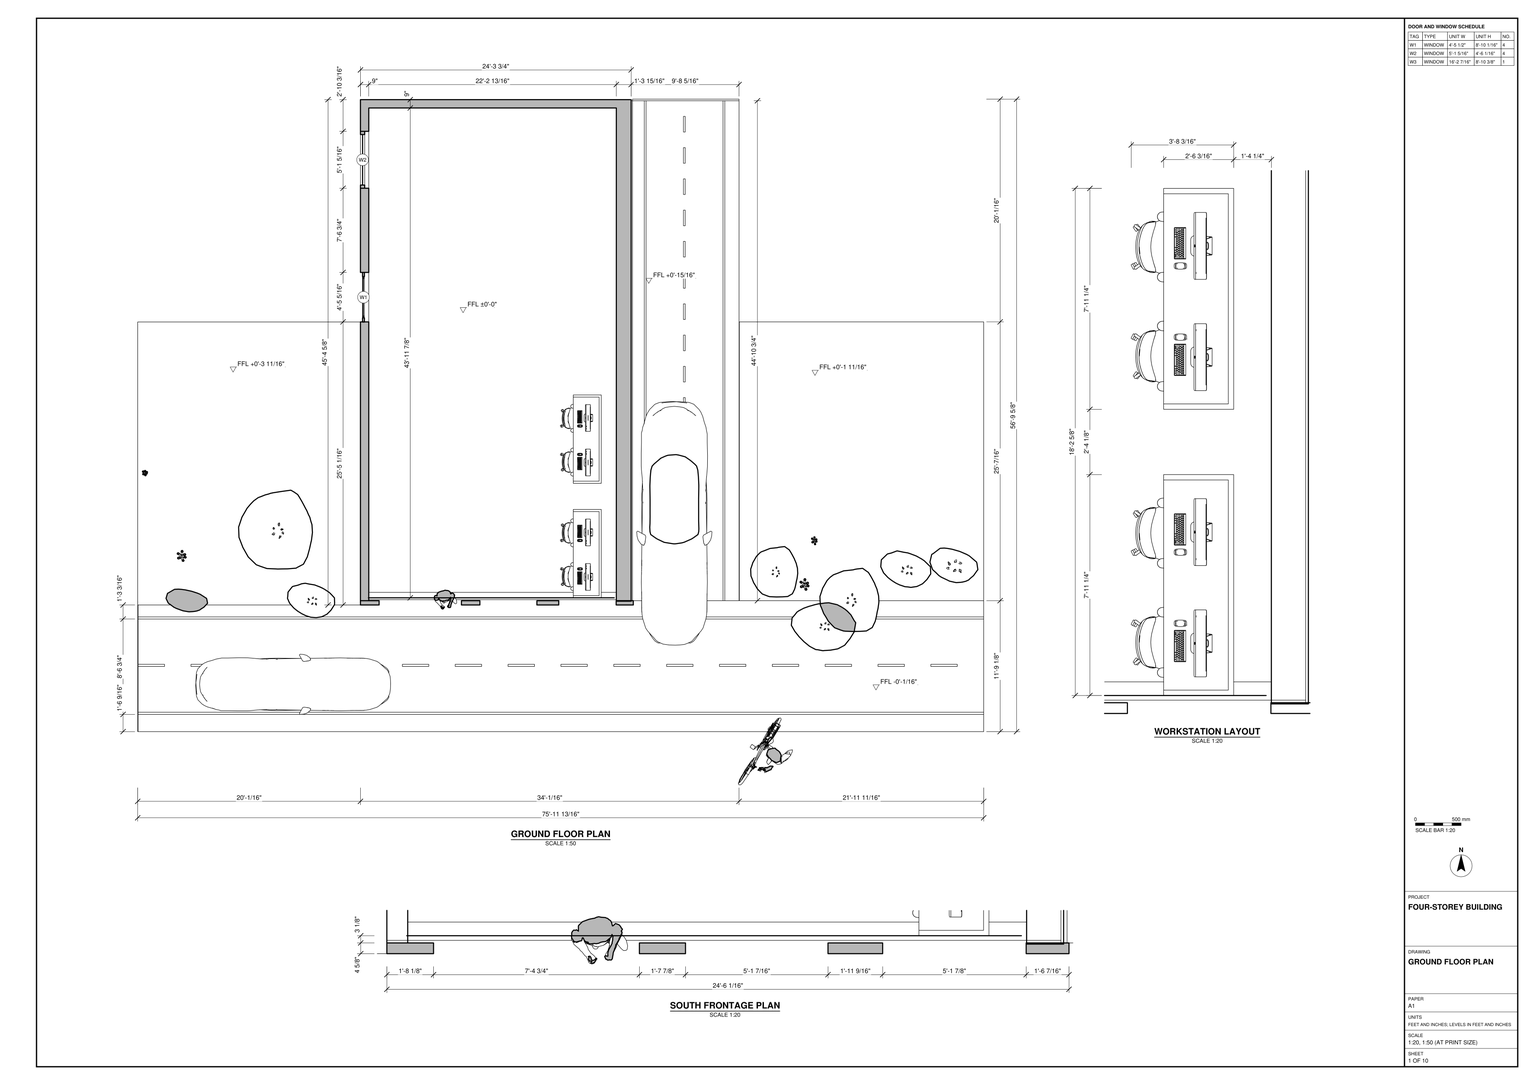
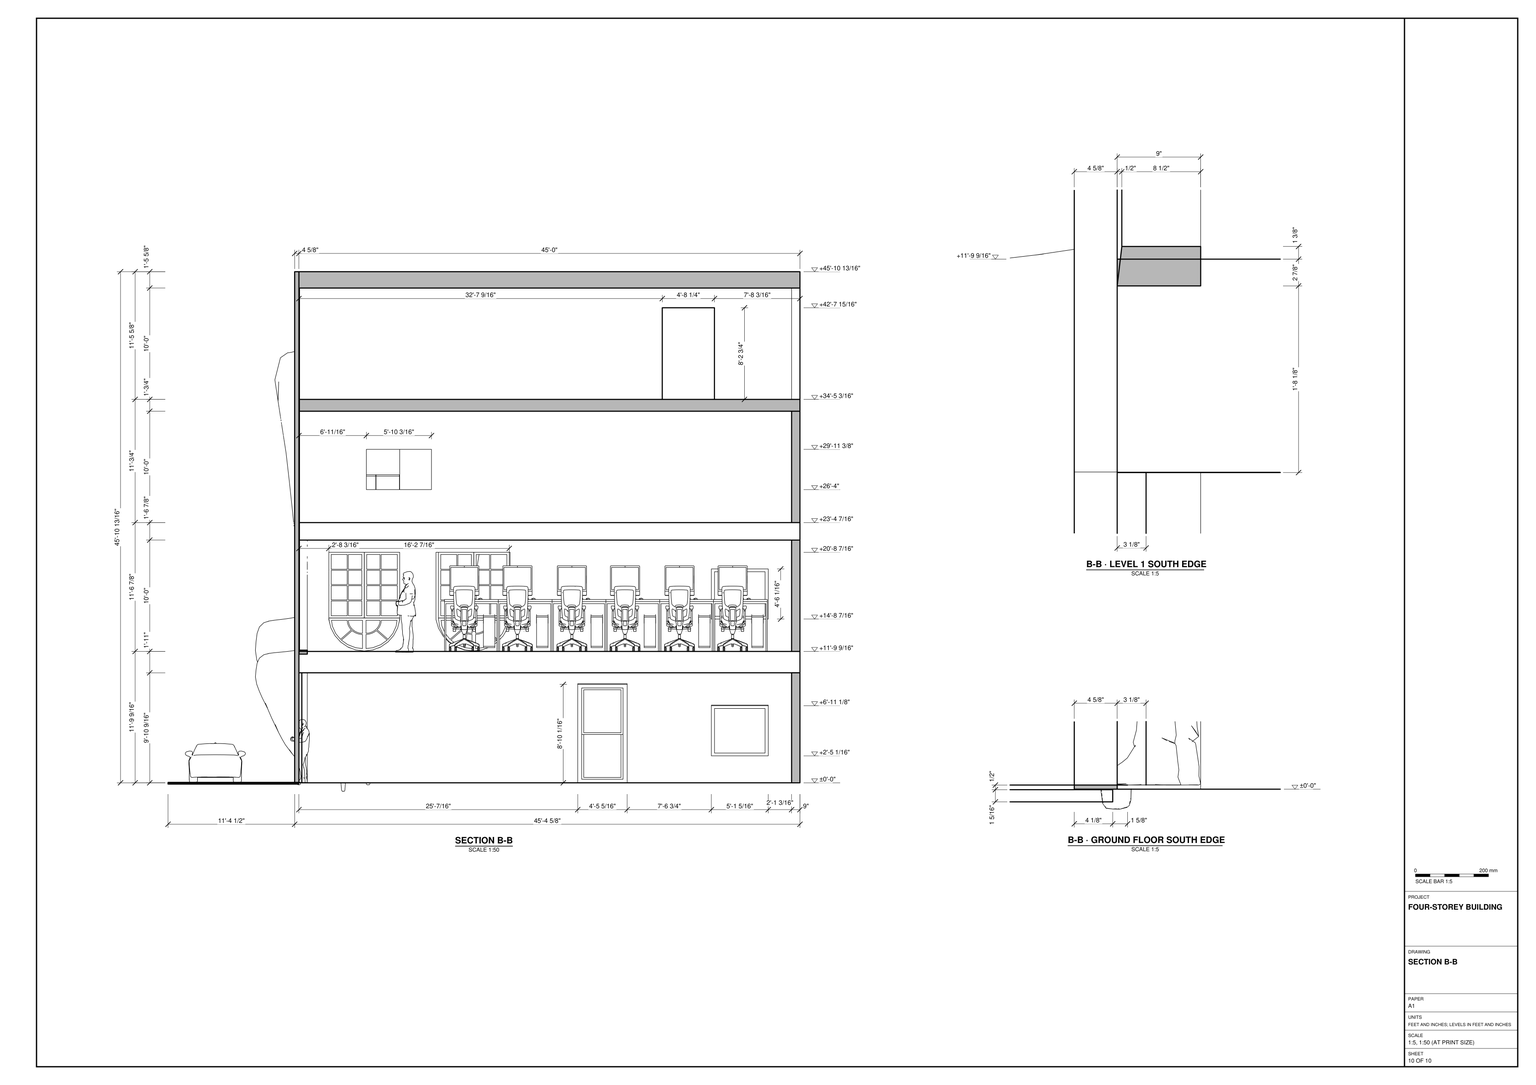
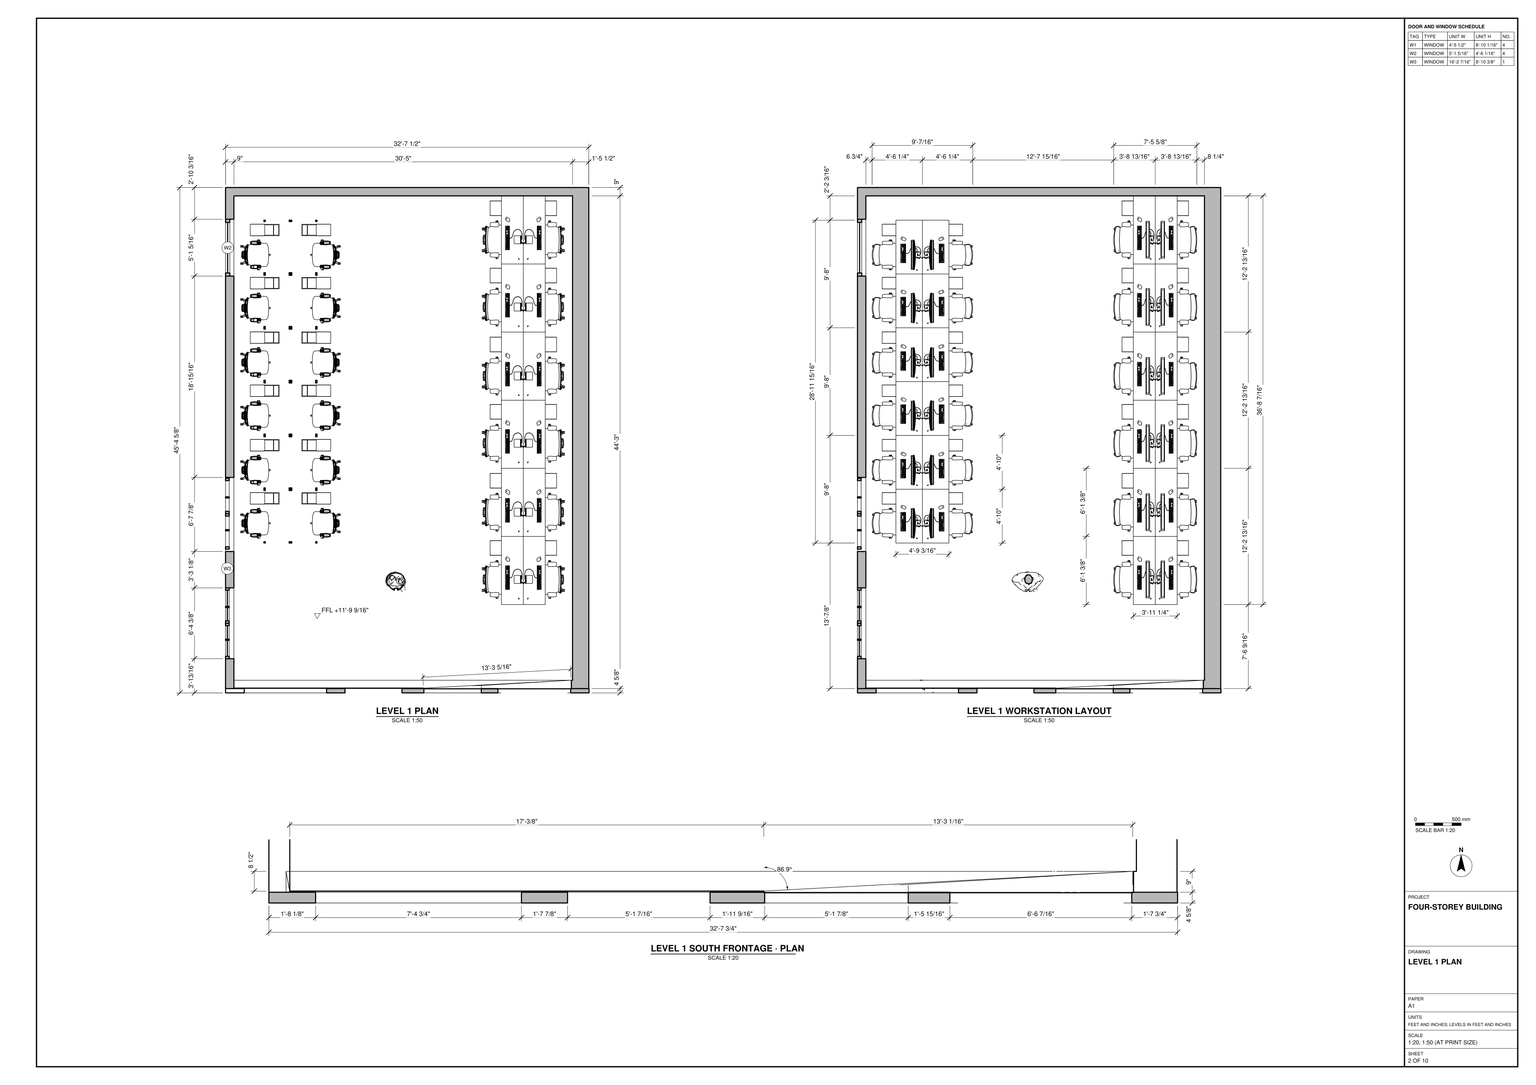
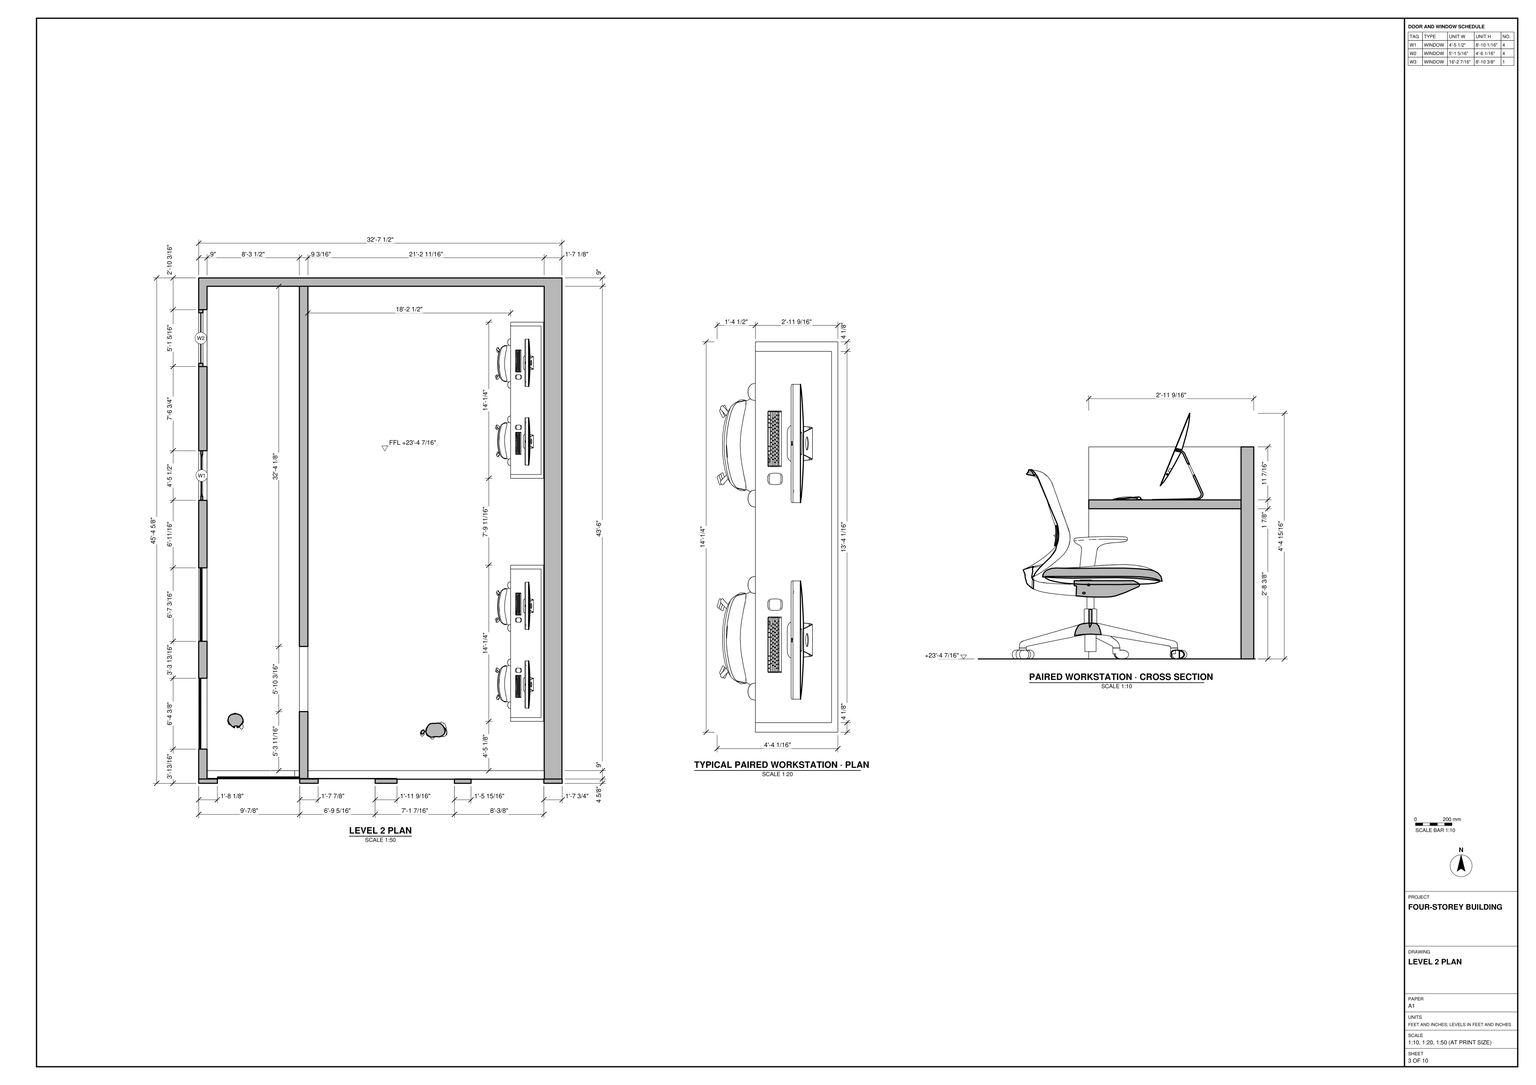
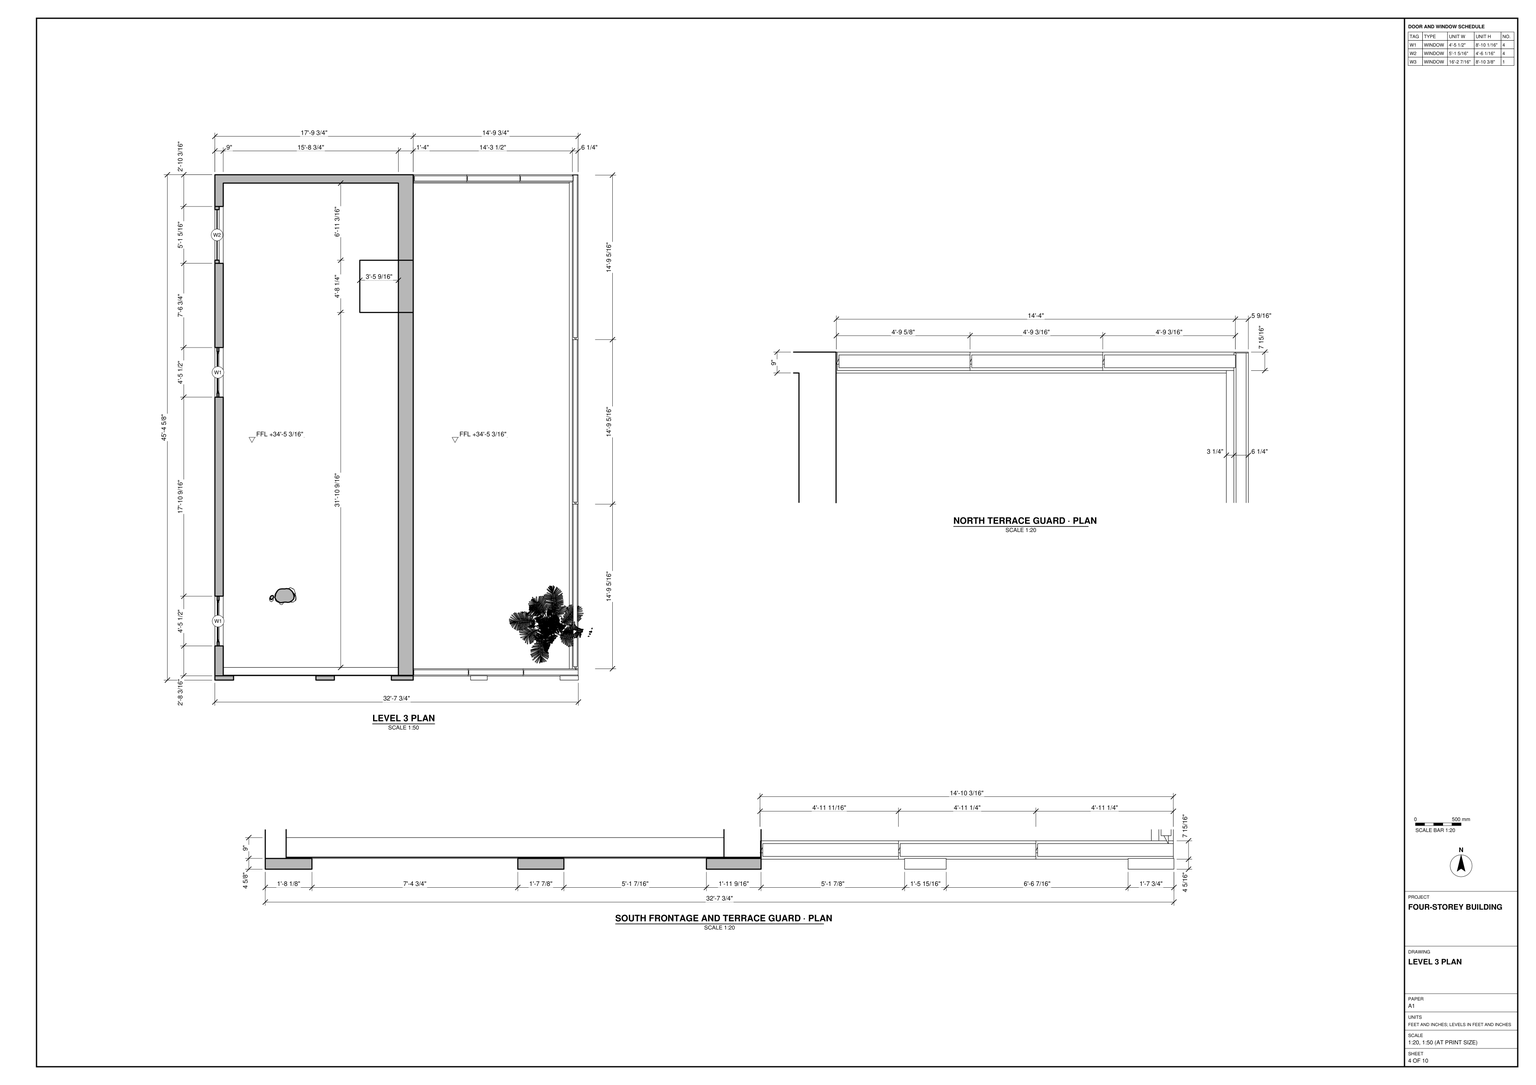
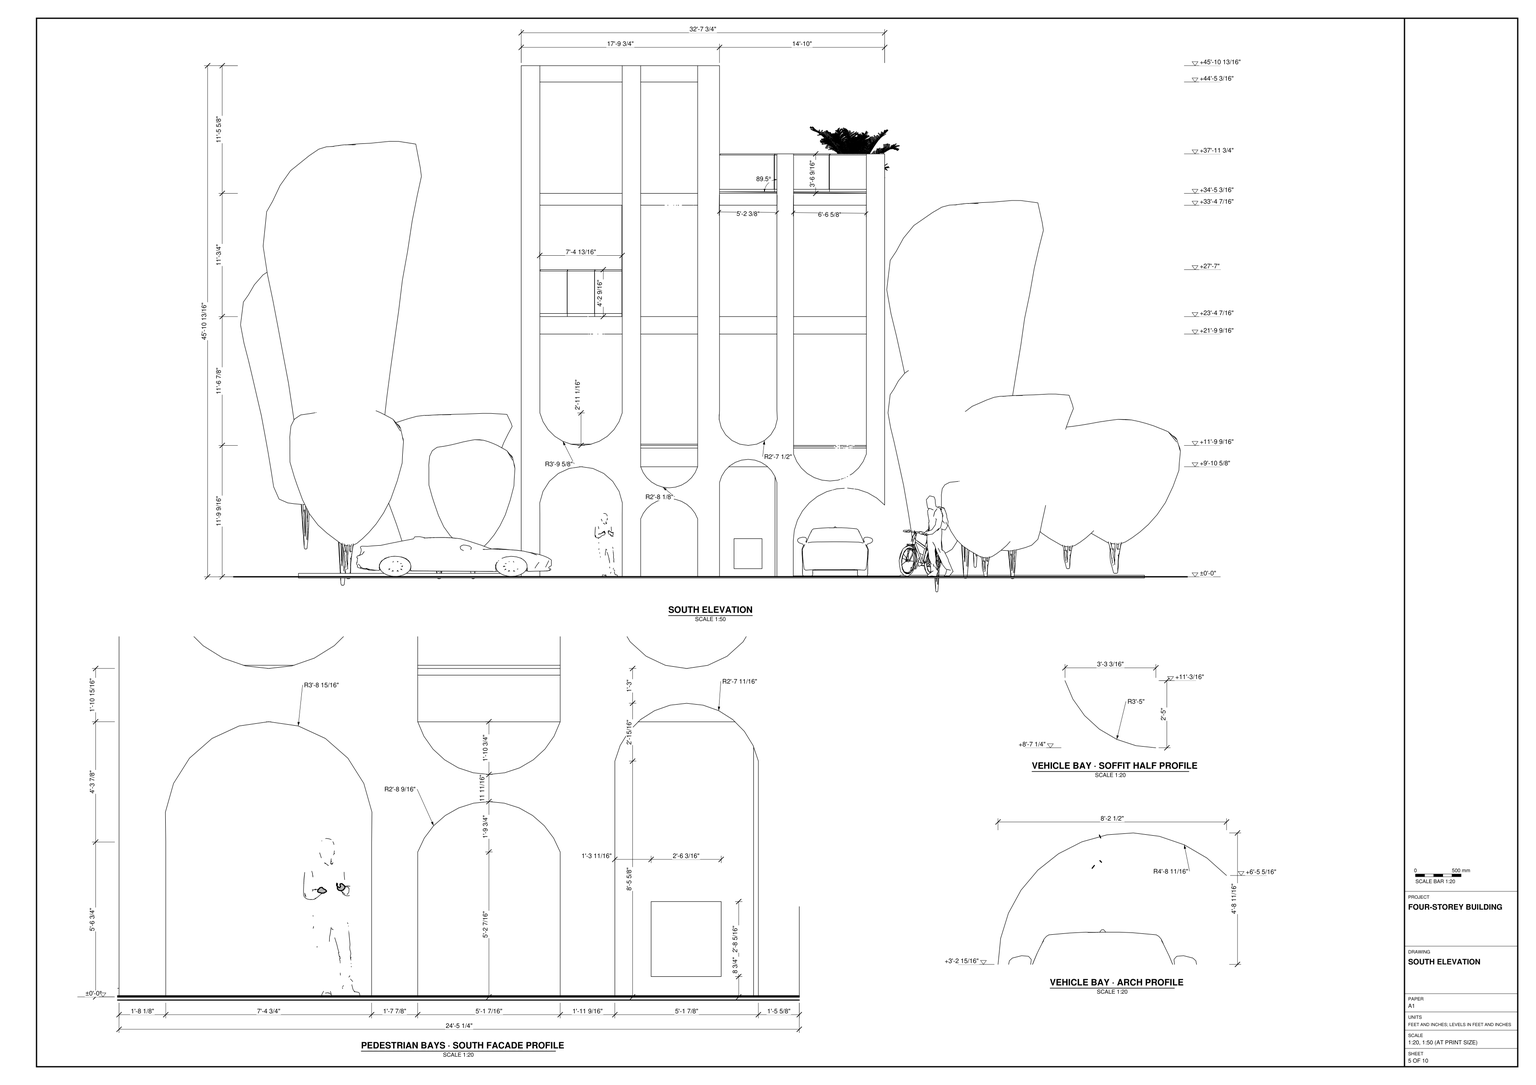
Build the four-storey office building and its site in SketchUp using task_files/diagram_01.pdf. Work in feet and inches. The overall model extents, including the site, are 84'-5" along X, 61'-7" along Y and 47'-3 1/16" along Z. Set the finished floor levels to ±0'-0", +11'-9 9/16", +23'-4 7/16" and +34'-5 3/16".

Lay out the street along the south frontage and the drive beside the narrower ground floor. Use the floor plans for the wall positions and thicknesses on each storey. Follow the sections for the floor slabs and flat roof, and use the frontage details to set the glazing and its vertical divisions relative to the slab edges. Place the window units in their scheduled openings. Include stairs and fixed joinery only where shown.

Size and position the ground-floor desks from the enlarged workstation layout. On the first upper floor, arrange the facing workstations in two banks with a clear aisle between them. Include the chairs and computer equipment shown at the desks. Place the vehicles and planting as shown on the site plan. Decor and loose items may be any suitable library components.

Keep shell elements such as walls, slabs and roof, and each furniture or joinery piece, in separate groups or components. Use components for repeated parts. Save one SketchUp model as output_files/four_storey_office_building_and_its_street_frontage.skp.

# SketchUp Ruby script. Lengths in inches.
U = 1.inch
M = Sketchup.active_model
def pt(a) = Geom::Point3d.new(a.map { |v| v * U })
def face(e, loops, mat)
  f = e.add_face(loops[0].map { |a| pt(a) })
  loops[1..].each { |l| e.add_face(l.map { |a| pt(a) }).erase! }
  f.material = f.back_material = mat if mat
  f
end
# faces: each face lists its corners as indices into pts; further lists are holes
def faces(e, pts, list, mat = nil) = list.each { |f| face(e, (f[0].is_a?(Array) ? f : [f]).map { |l| l.map { |i| pts[i] } }, mat) }
# xy, xz, yz: faces in a plane at the given z, y or x. An outline is a flat list of corners, or four numbers for a rectangle; further outlines are holes
def ring(l) = l.size == 4 ? [[l[0], l[1]], [l[2], l[1]], [l[2], l[3]], [l[0], l[3]]] : l.each_slice(2).to_a
def flat(e, list, mat, &to3) = list.each { |f| face(e, (f[0].is_a?(Array) ? f : [f]).map { |l| ring(l).map { |u, v| to3.(u, v) } }, mat) }
def xy(e, z, list, mat = nil) = flat(e, list, mat) { |x, y| [x, y, z] }
def xz(e, y, list, mat = nil) = flat(e, list, mat) { |x, z| [x, y, z] }
def yz(e, x, list, mat = nil) = flat(e, list, mat) { |y, z| [x, y, z] }
def lines(e, pts, list) = list.each { |a, b| e.add_line(pt(pts[a]), pt(pts[b])) }
# prism: a flat outline (further loops are holes) pulled along v
def prism(e, loops, v, mat = nil)
  f = face(e, loops, mat); d = Geom::Vector3d.new(v.map { |x| x * U })
  f.pushpull(f.normal.samedirection?(d) ? d.length : -d.length)
end
def box(e, o, s, mat = nil) = prism(e, [[o, [o[0] + s[0], o[1], o[2]], [o[0] + s[0], o[1] + s[1], o[2]], [o[0], o[1] + s[1], o[2]]]], [0, 0, s[2]], mat)
def at(x, y, z, deg = 0) = Geom::Transformation.translation(pt([x, y, z])) * Geom::Transformation.rotation(ORIGIN, Z_AXIS, deg.degrees)
def axes(o, x, y, z) = Geom::Transformation.new([*x, 0, *y, 0, *z, 0, *pt(o).to_a, 1])
def part(name) = M.definitions.add(name)
# library, detail: a bought-in or finely detailed component or shape, given as its bounding box
def library(name, o, s) = part(name).tap { |d| box(d.entities, o, s) }
def detail(e, o, s) = box(e.add_group.entities, o, s)
def put(e, d, t, mat = nil) = e.add_instance(d, t).tap { |i| i.material = mat if mat }
def group(e, t, mat = nil) = e.add_group.tap { |g| g.transformation = t; g.material = mat if mat }.entities
root = M.entities
M.materials.add("Aluminum_Anodized_Clear\#1").color = [178, 178, 174]
M.materials.add("Aluminum_Anodized_DarkGray\#1").color = [63, 63, 63]
M.materials.add("Bricks A04 100cm").color = [167, 128, 100]
M.materials.add("Concrete Grey 06 100cm").color = [123, 122, 117]
M.materials.add("Glass Clear 001").color = [0, 0, 0]
M.materials.add("Grass E 200cm\#1").color = [123, 134, 58]
M.materials.add("Windows").color = [58, 58, 58]
M.materials.add("[Asphalt_New]").color = [67, 60, 62]
M.materials.add("[Color_000]").color = [255, 255, 255]
M.materials.add("[Color_006]").color = [86, 86, 86]
M.materials.add("[Translucent Glass Gray]1").color = [128, 128, 128]
M.materials.add("[Translucent_Glass_Gray]").color = [128, 128, 128]
M.materials.add("[Translucent_Glass_Gray]1").color = [167, 187, 214]
M.materials.add("glass_architectural\#1").color = [217, 197, 188]
c1 = library("Schefflera arboricola 004",[-66.29,-60.4,-0.79],[131.92,126.97,148.56])
c2 = library("Schefflera arboricola 003",[-47.85,-46.83,-0.79],[92.88,94.95,107.86])
c3 = library("Car 034",[-40.54,-85.05,-1.09],[81.08,168.69,53.52])
c4 = part("Window+06")
g1 = group(c4.entities,at(-11,5.5,0,-90))
xy(g1,0,[[0,11,5.5,35]],"Windows")
xy(g1,2,[[0,13,5.5,33]],"Windows")
xy(g1,53,[[0,13,5.5,33]],"Windows")
xy(g1,55,[[0,11,5.5,35]],"Windows")
xz(g1,11,[[0,0,5.5,55]],"Windows")
xz(g1,13,[[0,2,5.5,53]],"Windows")
xz(g1,33,[[0,2,5.5,53]],"Windows")
xz(g1,35,[[0,0,5.5,55]],"Windows")
yz(g1,0,[[[11,0,35,55],[13,2,33,53]]],"Windows")
yz(g1,5.5,[[[11,0,35,55],[13,2,33,53]]],"Windows")
g2 = group(g1,at(2.75,2,2))
xy(g2,0,[[0,11,2,31]],"Windows")
xy(g2,1,[[0,12,1,30],[1,12,2,30]],"Windows")
xy(g2,25,[[0,12,1,30],[1,12,2,30]],"Windows")
xy(g2,26,[[0,11,2,31]],"Windows")
xz(g2,11,[[0,0,2,26]],"Windows")
xz(g2,12,[[0,1,1,25],[1,1,2,25]],"Windows")
xz(g2,30,[[0,1,1,25],[1,1,2,25]],"Windows")
xz(g2,31,[[0,0,2,26]],"Windows")
yz(g2,0,[[[11,0,31,26],[12,1,30,25]]],"Windows")
yz(g2,1,[[12,1,30,25]],"[Translucent Glass Gray]1")
yz(g2,2,[[[11,0,31,26],[12,1,30,25]]],"Windows")
g3 = group(g1,at(0.75,2,27))
xy(g3,0,[[0,11,2,31]],"Windows")
xy(g3,1,[[0,12,1,30],[1,12,2,30]],"Windows")
xy(g3,25,[[0,12,1,30],[1,12,2,30]],"Windows")
xy(g3,26,[[0,11,2,31]],"Windows")
xz(g3,11,[[0,0,2,26]],"Windows")
xz(g3,12,[[0,1,1,25],[1,1,2,25]],"Windows")
xz(g3,30,[[0,1,1,25],[1,1,2,25]],"Windows")
xz(g3,31,[[0,0,2,26]],"Windows")
yz(g3,0,[[[11,0,31,26],[12,1,30,25]]],"Windows")
yz(g3,1,[[12,1,30,25]],"[Translucent Glass Gray]1")
yz(g3,2,[[[11,0,31,26],[12,1,30,25]]],"Windows")
c5 = library("Group\#17",[0,0,0],[177.17,118.11,3.9375])
c6 = part("window+1")
g4 = group(c6.entities,at(0,0,177.17))
put(g4,c5,axes([0,0,0],[0,0,-1],[0,1,0],[1,0,0]))
g5 = group(g4,at(1.97,3.9375,-4.36),"[Translucent_Glass_Gray]")
yz(g5,0,[[0,-168.87,26.65,-142.34],[28.62,-168.87,51.08,-142.34],[59.15,-168.87,81.32,-142.34],[83.29,-168.87,110.24,-142.34],[0,-140.375,26.65,-114.83],
  [28.62,-140.375,51.08,-114.83],[59.15,-140.375,81.32,-114.83],[83.29,-140.375,110.24,-114.83],[0,-112.86,26.65,-87.32],[28.62,-112.86,51.08,-87.32],
  [59.15,-112.86,81.32,-87.32],[83.29,-112.86,110.24,-87.32],[0,-85.35,26.65,-58.83],[28.62,-85.35,51.08,-58.83],[59.15,-85.35,81.32,-58.83],
  [83.29,-85.35,110.24,-58.83],[0.55,-50.76,26.65,-50.76,26.93,-47.45,27.62,-44.2,28.72,-41.07,30.21,-38.1,32.07,-35.35,33.61,-33.59,15.58,-16.55,15.5625,-16.53,7.41,-27.15,1.91,-40.4375],[28.79,-50.76,52.17,-50.76,52.17,-27.38,50.2,-27.38,49.14,-27.47,46.14,-28.11,43.24,-29.125,40.5,-30.5,37.96,-32.22,35.65,-34.25,33.63,-36.55,31.91,-39.1,30.53,-41.84,29.52,-44.73,28.875,-47.74,28.79,-48.79],[58.07,-50.76,81.32,-50.76,81.32,-48.79,81.24,-47.74,80.61,-44.75,79.6,-41.87,78.24,-39.14,76.53,-36.61,74.52,-34.3125,72.22,-32.3,69.6875,-30.59,66.96,-29.22,64.08,-28.22,61.09,-27.59,60.04,-27.51,58.07,-27.51],[83.45,-50.76,109.68,-50.76,108.33,-40.4375,102.82,-27.15,94.67,-16.53,76.5625,-33.66,78.09,-35.4,79.94,-38.15,81.42,-41.1,82.51,-44.23,83.19,-47.46],
  [75.17,-32.27,93.28,-15.14,82.66,-6.99,69.375,-1.49,58.07,0,58.07,-25.38,61.37,-25.64,64.6,-26.32,67.73,-27.41,70.68,-28.89,73.43,-30.74],[35,-32.2,36.75,-30.66,39.51,-28.8,42.47,-27.31,45.61,-26.21,48.86,-25.52,52.17,-25.25,52.17,0,40.86,-1.49,27.58,-6.99,16.96,-15.14]])
put(g4,c5,axes([0,182.58,0],[0,0,-1],[0,1,0],[1,0,0]))
c7 = part("GLASS")
prism(c7.entities,[[[48,0,0],[0,0,0],[0,0.8,0],[48.96,0.8,0]]],[0,0,36])
c8 = part("STEEL BAR")
box(c8.entities,[0,-0.1,0],[48,1.8,1.2])
c9 = part("LOWER PART")
box(c9.entities,[0,-0.6,0],[48.6,2.6,2.6])
c10 = part("BALCONY GLASS ")
put(c10.entities,c7,at(0,0.9,2.6),"glass_architectural\#1")
put(c10.entities,c8,at(0,0.5,38.6),"Aluminum_Anodized_DarkGray\#1")
put(c10.entities,c9,at(0,0.6,0),"Aluminum_Anodized_Clear\#1")
c11 = part("NO 3")
put(c11.entities,c10,at(0,0,0))
put(c11.entities,c10,at(48.6,0,0))
put(c11.entities,c10,at(97.2,0,0))
c12 = part("BIC_Bike Shop - Window - Small")
xy(c12.entities,-8,[[[0,0,36,36],[2,2,34,34]]],"[Color_006]")
xy(c12.entities,-4,[[2,2,34,34]],"[Translucent_Glass_Gray]1")
xy(c12.entities,0,[[[0,0,36,36],[2,2,34,34]]],"[Color_006]")
xz(c12.entities,0,[[0,-8,36,0]],"[Color_006]")
xz(c12.entities,2,[[2,-8,34,-4],[2,-4,34,0]],"[Color_006]")
xz(c12.entities,34,[[2,-8,34,-4],[2,-4,34,0]],"[Color_006]")
xz(c12.entities,36,[[0,-8,36,0]],"[Color_006]")
yz(c12.entities,0,[[0,-8,36,0]],"[Color_006]")
yz(c12.entities,2,[[2,-8,34,-4],[2,-4,34,0]],"[Color_006]")
yz(c12.entities,34,[[2,-8,34,-4],[2,-4,34,0]],"[Color_006]")
yz(c12.entities,36,[[0,-8,36,0]],"[Color_006]")
c13 = part("Untitled (6)")
xy(c13.entities,0,[[-437.53,-1998.08,-389.53,356.87],[[-383.53,-1998.08,-383.53,356.87,-256.03,356.87,-256.03,283.28,-250.03,283.28,-250.03,356.87,-124.03,356.87,-124.03,-1998.08],[-256.03,136.09,-250.03,209.6875],[-256.03,-158.28,-250.03,-84.68],[-256.03,-599.83,-250.03,-526.24],[-256.03,-11.09,-250.03,62.5],[-256.03,-452.64,-250.03,-379.05],[-256.03,-747.01,-250.03,-673.42],[-256.03,-305.46,-250.03,-231.87],[-256.03,-1630.12,-250.03,-1556.53],[-256.03,-1482.93,-250.03,-1409.34],[-256.03,-1335.75,-250.03,-1262.16],[-256.03,-894.2,-250.03,-820.6],[-256.03,-1924.49,-250.03,-1850.89],[-256.03,-1188.57,-250.03,-1114.97],[-256.03,-1777.3,-250.03,-1703.71],[-256.03,-1041.38,-250.03,-967.79]],[-118.03,-1998.08,-70.03,356.87]],"[Asphalt_New]")
xy(c13.entities,0,[[-389.53,-1998.08,-383.53,356.87],[-124.03,-1998.08,-118.03,356.87],[-256.03,-1924.49,-250.03,-1850.89],[-256.03,-1777.3,-250.03,-1703.71],[-256.03,-1630.12,-250.03,-1556.53],
  [-256.03,-1482.93,-250.03,-1409.34],[-256.03,-1335.75,-250.03,-1262.16],[-256.03,-1188.57,-250.03,-1114.97],[-256.03,-1041.38,-250.03,-967.79],[-256.03,-894.2,-250.03,-820.6],
  [-256.03,-747.01,-250.03,-673.42],[-256.03,-599.83,-250.03,-526.24],[-256.03,-452.64,-250.03,-379.05],[-256.03,-305.46,-250.03,-231.87],[-256.03,-158.28,-250.03,-84.68],
  [-256.03,-11.09,-250.03,62.5],[-256.03,136.09,-250.03,209.6875],[-256.03,283.28,-250.03,356.87]],"[Color_000]")
c14 = library("Group\#170",[0,0,-0.09],[44.81,94.49,48.85])
c15 = library("Group\#172",[0,0,-0.09],[44.81,94.49,48.85])
c16 = part("Office workstation bank")
put(c16.entities,c14,at(188.98,44.81,0.09,-90))
put(c16.entities,c15,axes([0,44.81,0.09],[0,1,0],[1,0,0],[0,0,1]))
put(c16.entities,c15,axes([188.98,44.81,0.09],[0,1,0],[1,0,0],[0,0,1]))
put(c16.entities,c14,at(0,44.81,0.09,-90))
put(c16.entities,c14,at(94.49,44.81,0.09,-90))
put(c16.entities,c15,axes([94.49,44.81,0.09],[0,1,0],[1,0,0],[0,0,1]))
c17 = library("Reception desk",[23.57,0,0],[37.45,80.71,54.72])
c18 = library("Tariq 001 Standing",[-13.52,-8.8,0],[27.07,17.52,69.71])
c19 = library("Hugh 001 Standing",[-12.24,-10.14,0],[24.44,20.33,67.86])
c20 = library("Katja 001 Standing",[-10.51,-13.65,0],[20.97,27.3,64.32])
c21 = library("Jalen Walking 001",[-18.74,-36.02,0],[37.48,72.04,73.58])
c22 = library("Untitled+(35)",[-36.2,-34.81,25.37],[51.5,58.42,71.3])
c23 = library("Palmilla",[-52.93,-43.2,-6.65],[96.66,94.88,84.22])
c24 = library("Dome Light",[-12,-12,0],[24,24,12])
c25 = library("Dome Light\#1",[-12,-12,0],[24,24,12])
c26 = library("Group\#2",[-859.75,865.09,0],[391.75,7.56,550.82])
box(root,[0,136.48,1.37],[240.0625,305,3.69],"Grass E 200cm\#1")
box(root,[0.02,0,0],[911.79,140.625,1.3125])
box(root,[396.25,532.6875,414.5625],[57.5625,56.26,98.76])
xy(root,1.37,[[533.3125,141.11,648.125,681.61],[648.125,141.11,648.4375,441.57]])
xy(root,1.37,[[648.4375,141.11,911.8125,441.57]],"Grass E 200cm\#1")
xy(root,2.31,[[533.3125,141.11,648.125,681.61]])
xy(root,3.06,[[648.4375,141.11,911.8125,441.57]],"Grass E 200cm\#1")
xy(root,140.05,[[247.44,141.11,612.5,150.11]],"Glass Clear 001")
xy(root,144.3,[[249.0625,141.61,453.45,141.61,612.5,150.11,247.44,150.11]],"Glass Clear 001")
xy(root,281.8125,[[240.0625,289.51,249.0625,368.7]])
xy(root,282.82,[[240.0625,173.32,249.0625,249.35]],"Concrete Grey 06 100cm")
xy(root,283.0625,[[240.0625,289.51,249.0625,368.7]])
xy(root,414.5625,[[631.5625,141.11,622.08,148.73,631.5625,148.73]])
xy(root,416.25,[[453.5,141.11,631.5625,148.73]])
xy(root,534.5625,[[249.0625,141.11,453.45,141.61]],"Glass Clear 001")
xz(root,140.88,[[453.5,141.73,612.5,401.8125]],"Glass Clear 001")
xz(root,141.11,[[533.3125,1.37,648.125,2.31]])
xz(root,141.11,[[631.5625,414.5625,631.5625,416.25,453.5,416.25]],"Concrete Grey 06 100cm")
xz(root,141.11,[[247.44,140.05,249.0625,140.05,247.44,144.3]],"Glass Clear 001")
xz(root,141.61,[[249.0625,144.3,453.45,534.5625]],"Glass Clear 001")
xz(root,144.22,[[248.63,1.8125,513.625,119.9375]],"Glass Clear 001")
xz(root,148.73,[[453.5,414.5625,453.5,416.25,622.08,416.25,622.08,414.93,631.5625,414.93,631.5625,414.5625],[622.08,414.5625,631.5625,414.93],[622.08,414.93,631.5625,415.0625],[622.08,415.0625,631.5625,416.25],[622.08,415.0625,631.5625,416.25]])
xz(root,150.11,[[247.44,140.05,612.5,144.3]],"Glass Clear 001")
xz(root,289.51,[[240.0625,281.8125,249.0625,283.0625]])
xz(root,368.7,[[240.0625,281.8125,249.0625,283.0625]])
xz(root,441.57,[[648.4375,1.37,911.8125,3.06]],"Grass E 200cm\#1")
xz(root,672.07,[[453.82,413.7,622.08,414.65,622.08,415.52,453.8125,414.58]])
xz(root,681.11,[[622.08,413.82,631.5625,415.51],[622.08,414.63,622.08,415.51,622.08,414.64]])
xz(root,681.61,[[533.3125,1.37,648.125,2.31]])
yz(root,240.0625,[[173.32,281.8125,173.32,282.82,249.35,282.82,252.52,281.8125],[289.51,281.8125,368.7,283.0625]],"Concrete Grey 06 100cm")
yz(root,247.44,[[141.11,140.05,150.11,144.3]],"Glass Clear 001")
yz(root,249.0625,[[289.51,281.8125,368.7,283.0625]])
yz(root,249.0625,[[141.11,140.05,141.11,534.5625,141.61,534.5625,141.61,144.3]],"Glass Clear 001")
yz(root,453.45,[[141.11,140.05,141.61,144.3,141.61,534.5625,141.11,534.5625]],"Glass Clear 001")
yz(root,453.5,[[140.88,401.8125,141.11,416.25,148.73,416.25,148.73,414.5625]])
yz(root,533.3125,[[141.11,1.37,681.61,2.31]])
yz(root,612.5,[[141.11,140.05,150.11,140.05,150.11,144.3,140.88,141.73]],"Glass Clear 001")
yz(root,622.08,[[681.11,413.82,148.73,414.5625,148.73,416.25,672.07,415.52,680.23,415.51,681.11,415.51],[680.23,414.64,680.23,415.51,672.07,415.52,672.07,414.65],[680.23,414.64,681.11,415.51]])
yz(root,631.5625,[[681.11,413.82,681.11,415.51,148.73,416.25,148.73,414.5625],[141.11,414.5625,148.73,416.25]],"Concrete Grey 06 100cm")
yz(root,648.125,[[141.11,1.37,681.61,2.31]])
yz(root,648.4375,[[141.11,1.37,441.57,3.06]],"Grass E 200cm\#1")
# 1 loose lines left out
p = [[453.45,141.11,140.05],[453.5,140.88,141.73],[453.45,141.61,144.3],[453.5,141.11,140.05],[612.5,141.11,140.05],[612.5,140.88,141.73],
  [247.44,141.11,144.3],[249.0625,141.11,140.05],[247.44,150.11,144.3],[249.0625,141.61,144.3],[612.5,150.11,144.3],[453.5,140.88,401.8125],
  [453.5,148.73,414.5625],[622.08,148.73,414.5625],[612.5,140.88,401.8125],[622.08,672.07,414.65],[453.82,672.07,413.7],[453.82,681.1,413.6875],
  [622.08,681.11,414.63],[622.08,681.11,414.64],[622.08,680.23,414.64],[453.8125,672.07,414.58],[453.8125,681.11,414.5625],[622.08,681.11,415.51],
  [622.08,681.11,413.82],[631.5625,681.11,413.82],[631.5625,148.73,414.5625],[622.08,672.07,415.52],[622.08,680.23,415.51],[622.08,148.73,416.25],
  [631.5625,148.73,416.25],[631.5625,681.11,415.51]]
faces(root,p,[[0,1,2],[1,0,3],[3,4,5,1],[6,7,8],[9,8,7],[0,2,9,7],[1,10,2],[5,10,1]],"Glass Clear 001")
faces(root,p,[[11,12,13,14],[15,16,17,18,19,20],[21,22,17,16],[22,23,18,17],[13,24,25,26],[21,27,28,23,22],[28,27,29,30,31,23]])
put(root,c1,axes([7.82,278.72,32.9375],[1.06,0,0],[0,1,0],[0,0,2.1296]))
put(root,c1,axes([151.57,215.65,0.16],[1.2,0,0],[0,1.2,0],[0,0,1.2]))
put(root,c1,axes([718.9,158.02,1.8125],[1.28,0,0],[0,1.28,0],[0,0,2.74138]))
put(root,c1,axes([769.6,141.11,0.27],[1,0,0],[0,1,0],[0,0,1.34]))
put(root,c2,axes([53.78,141.01,0.58],[1.32,0,0],[0,1,0],[0,0,1.73203]))
put(root,c2,axes([188.3,141.01,0.31],[1,0,0],[0,1,0],[0,0,1.39]))
put(root,c2,at(740.74,113.62,2))
put(root,c2,axes([829.43,174.43,11],[1.15,0,0],[0,1.15,0],[0,0,1.15]))
put(root,c1,axes([729.37,205.53,13.51],[0.88,0,0],[0,1,0],[0,0,2.5311]))
put(root,c3,axes([578.39,225.59,2.9],[1,0,0],[0,1.5568,0],[0,0,1]))
put(root,c1,axes([47.65,188.84,-5.3],[1.2932,0,0],[0,1.22,0],[0,0,3.2208]))
put(root,c2,axes([880.67,178.68,6.27],[1.5525,0,0],[0,1.5525,0],[0,0,1.53883]))
put(root,c4,axes([242.3125,494.89,281.8125],[0,-2.22917,0],[0.375,0,0],[0,0,1.92841]))
put(root,c6,axes([244,173.32,249.8125],[-1,0,0],[0,0.64664,0],[0,0,-0.60043]))
put(root,c4,axes([242.3125,494.89,414.5625],[0,-2.22917,0],[0.375,0,0],[0,0,1.92841]))
put(root,c4,axes([242.3125,494.89,1.37],[0,-2.22917,0],[0.375,0,0],[0,0,1.92841]))
put(root,c4,axes([242.5,226.82,414.5625],[0,-2.22917,0],[0.375,0,0],[0,0,1.92841]))
put(root,c11,axes([631.5625,148.73,416.25],[-1.21914,0,0],[0,-3.0602,0],[0,0,1.0272]))
put(root,c11,axes([242.66,173.32,282.82],[0,0.52383,0],[-1,0,0],[0,0,1.27]))
put(root,c11,axes([243.98,289.51,283.0625],[0,0.54268,0],[-1,0,0],[0,0,1.27]))
put(root,c12,axes([240.0625,646.92,177.83],[0,-1.70312,0],[0,0,1.50107],[-0.5763,0,0]))
put(root,c12,axes([240.0625,646.92,448.7],[0,-1.70312,0],[0,0,1.50107],[-0.5763,0,0]))
put(root,c12,axes([240.0625,646.92,30.4375],[0,-1.70312,0],[0,0,1.50107],[-0.5763,0,0]))
put(root,c12,axes([240.0625,646.92,316.58],[0,-1.70312,0],[0,0,1.50107],[-0.5763,0,0]))
put(root,c13,axes([508.3,222.75,2.31],[-0.31958,0,0],[0,-0.22878,0],[0,0,0.279]))
put(root,c13,axes([138.56,169.33,1.8125],[0,0.387,0],[-0.387,0,0],[0,0,0.387]))
put(root,c11,axes([625.3,680.71,415.51],[0,-3.6487,0],[2.4075,0,0],[0,0,1.07]))
put(root,c11,axes([625.98,681.11,414.5625],[-1.177,0,0],[0,-3.0602,0],[0,0,1.07]))
put(root,c16,axes([516.21,672.11,142.85],[0,-1.55368,0],[1,0,0],[0,0,1.5]))
put(root,c16,axes([255.82,645.9,142.9375],[0,-1.22741,0],[1.21,0,0],[0,0,1.89]))
put(root,c17,axes([427.63,144.22,10.13],[1.18,0,0],[0,1.18,0],[0,0,0.6844]))
put(root,c17,axes([526.98,203.22,281.8125],[1.39,0,0],[0,2.085,0],[0,0,0.96744]))
put(root,c17,axes([526.98,465.16,281.8125],[1.39,0,0],[0,2.085,0],[0,0,0.96744]))
put(root,c17,axes([427.63,267.59,10.13],[1.18,0,0],[0,1.18,0],[0,0,0.6844]))
put(root,c3,axes([166.68,51.01,2.6875],[0,0.8,0],[-1.24544,0,0],[0,0,0.8]))
put(root,c18,at(279.875,203.41,291.03))
put(root,c18,axes([423.48,256.09,142.06],[1.25,0,0],[0,1.25,0],[0,0,1.25]))
put(root,c19,at(331.68,142.22,1.8125))
put(root,c20,axes([493.89,183.04,281.8125],[1.43,0,0],[0,1.43,0],[0,0,1.43]))
put(root,c21,axes([678.13,-25.75,1.8125],[1.02191,-0.59,0],[0.59,1.02191,0],[0,0,1.18]))
put(root,c20,axes([313.79,216.76,414.5625],[1.43,0,0],[0,1.43,0],[0,0,1.43]))
put(root,c22,at(594.36,146.97,55.58))
put(root,c23,at(604.06,186.73,408.9))
put(root,c22,at(327.84,151.59,191.76))
put(root,c22,at(410.95,147.59,321.35))
put(root,c1,axes([688.01,171.53,-13.56],[0.7936,0,0],[0,0.7936,0],[0,0,1.69965]))
put(root,c11,axes([348.8125,143.71,281.8125],[-0.60765,0,0],[0,-1,0],[0,0,1.27]))
put(root,c24,at(560.9,145.76,232.72))
put(root,c25,at(560.23,140.88,378.76))
put(root,c24,at(399.53,136.48,70.56))
g6 = group(root,at(-660.5625,139.09,143))
box(g6,[900.625,2.02,119.9375],[391.5,540,18.875],"Concrete Grey 06 100cm")
box(g6,[900.625,2.02,258.8125],[391.5,540,12.75],"Concrete Grey 06 100cm")
xy(g6,-39.4375,[[1193.07,2.02,1275.63,5.83]],"Concrete Grey 06 100cm")
xy(g6,-23.0625,[[900.625,2.02,900.625,542.02,1292.125,542.02,1292.125,2.02,1275.63,2.02,1275.63,5.83,1193.07,5.83,1193.07,2.02]],"Concrete Grey 06 100cm")
xy(g6,-0.0625,[[900.625,2.02,1292.125,542.02]],"Concrete Grey 06 100cm")
xz(g6,2.02,[[1193.07,-39.4375,1275.63,-39.4375,1275.63,-23.0625,1292.125,-23.0625,1292.125,-0.0625,900.625,-0.0625,900.625,-23.0625,1193.07,-23.0625]],"Concrete Grey 06 100cm")
xz(g6,5.83,[[1193.07,-39.4375,1275.63,-23.0625]],"Concrete Grey 06 100cm")
xz(g6,542.02,[[900.625,-23.0625,1292.125,-0.0625]],"Concrete Grey 06 100cm")
yz(g6,900.625,[[2.02,-23.0625,542.02,-0.0625]],"Concrete Grey 06 100cm")
yz(g6,1193.07,[[2.02,-39.4375,5.83,-23.0625]],"Concrete Grey 06 100cm")
yz(g6,1275.63,[[2.02,-39.4375,5.83,-23.0625]],"Concrete Grey 06 100cm")
yz(g6,1292.125,[[2.02,-23.0625,542.02,-0.0625]],"Concrete Grey 06 100cm")
g7 = group(root,at(-656.73,139.09,410))
xy(g7,4.5625,[[896.79,2.02,905.79,34.24],[1094.55,2.08,1094.55,533.02,905.79,533.02,905.79,355.8,896.79,355.8,896.79,542.02,1110.54,542.02,1110.54,2.08],[905.79,11.02,1094.55,533.02],[896.79,87.86,905.79,302.3]],"Bricks A04 100cm")
xy(g7,38.7,[[896.79,446.52,905.79,507.83]],"Bricks A04 100cm")
xy(g7,92.74,[[896.79,446.52,905.79,507.83]],"Bricks A04 100cm")
xy(g7,108.5,[[896.79,34.24,905.79,87.86],[896.79,302.3,905.79,355.8]],"Bricks A04 100cm")
xy(g7,124.5625,[[896.79,2.02,905.79,2.02,905.79,533.02,1094.55,533.02,1094.55,2.08,1110.54,2.08,1110.54,542.02,896.79,542.02]],"Bricks A04 100cm")
xz(g7,2.02,[[896.79,4.5625,905.79,124.5625]],"Bricks A04 100cm")
xz(g7,2.08,[[1094.55,4.5625,1110.54,124.5625]],"Bricks A04 100cm")
xz(g7,34.24,[[896.79,4.5625,905.79,108.5]],"Bricks A04 100cm")
xz(g7,87.86,[[896.79,4.5625,905.79,108.5]],"Bricks A04 100cm")
xz(g7,302.3,[[896.79,4.5625,905.79,108.5]],"Bricks A04 100cm")
xz(g7,355.8,[[896.79,4.5625,905.79,108.5]],"Bricks A04 100cm")
xz(g7,446.52,[[896.79,38.7,905.79,92.74]],"Bricks A04 100cm")
xz(g7,507.83,[[896.79,38.7,905.79,92.74]],"Bricks A04 100cm")
xz(g7,533.02,[[905.79,4.5625,1094.55,124.5625]],"Bricks A04 100cm")
xz(g7,542.02,[[896.79,4.5625,1110.54,124.5625]],"Bricks A04 100cm")
yz(g7,896.79,[[[2.02,4.5625,2.02,124.5625,542.02,124.5625,542.02,4.5625,355.8,4.5625,355.8,108.5,302.3,108.5,302.3,4.5625,87.86,4.5625,87.86,108.5,34.24,108.5,34.24,4.5625],[446.52,38.7,507.83,92.74]]],"Bricks A04 100cm")
yz(g7,905.79,[[2.02,4.5625,11.02,124.5625],[[11.02,4.5625,34.24,4.5625,34.24,108.5,87.86,108.5,87.86,4.5625,302.3,4.5625,302.3,108.5,355.8,108.5,355.8,4.5625,533.02,4.5625,533.02,124.5625,11.02,124.5625],[446.52,38.7,507.83,92.74]]],"Bricks A04 100cm")
yz(g7,1094.55,[[2.08,4.5625,533.02,124.5625]],"Bricks A04 100cm")
yz(g7,1110.54,[[2.08,4.5625,542.02,124.5625]],"Bricks A04 100cm")
g8 = group(root,at(-660.5625,139.09,531.125))
g9 = group(g8,at(315.95,2.02,-23.99))
box(g9,[584.68,0,27.43],[213.75,540,17.62],"Concrete Grey 06 100cm")
g10 = group(root,at(138.3125,141.11,0))
xy(g10,1.37,[[377.5625,-0.5,377.5625,531,110.75,531,110.75,353.78,101.75,353.78,101.75,540,393.52,540,393.52,-0.5],[101.75,0,110.75,300.47],[110.75,0,377.5625,9],[110.75,9,377.5625,531]],"Bricks A04 100cm")
xy(g10,30.4375,[[101.75,444.5,110.75,505.8125]],"Bricks A04 100cm")
xy(g10,85.12,[[101.75,444.5,110.75,505.8125]],"Bricks A04 100cm")
xy(g10,108.18,[[101.75,300.47,110.75,353.78]],"Bricks A04 100cm")
xy(g10,119.99,[[377.5625,-0.5,393.52,-0.5,393.52,540,101.75,540,101.75,0,110.75,0,110.75,531,377.5625,531]],"Bricks A04 100cm")
xz(g10,-0.5,[[377.5625,1.37,393.52,119.99]],"Bricks A04 100cm")
xz(g10,0,[[101.75,1.37,110.75,119.99]],"Bricks A04 100cm")
xz(g10,300.47,[[101.75,1.37,110.75,108.18]],"Bricks A04 100cm")
xz(g10,353.78,[[101.75,1.37,110.75,108.18]],"Bricks A04 100cm")
xz(g10,444.5,[[101.75,30.4375,110.75,85.12]],"Bricks A04 100cm")
xz(g10,505.8125,[[101.75,30.4375,110.75,85.12]],"Bricks A04 100cm")
xz(g10,531,[[110.75,1.37,377.5625,119.99]],"Bricks A04 100cm")
xz(g10,540,[[101.75,1.37,393.52,119.99]],"Bricks A04 100cm")
yz(g10,101.75,[[[0,1.37,0,119.99,540,119.99,540,1.37,353.78,1.37,353.78,108.18,300.47,108.18,300.47,1.37],[444.5,30.4375,505.8125,85.12]]],"Bricks A04 100cm")
yz(g10,110.75,[[0,1.37,9,119.99],[[9,1.37,300.47,1.37,300.47,108.18,353.78,108.18,353.78,1.37,531,1.37,531,119.99,9,119.99],[444.5,30.4375,505.8125,85.12]]],"Bricks A04 100cm")
yz(g10,377.5625,[[-0.5,1.37,531,119.99]],"Bricks A04 100cm")
yz(g10,393.52,[[-0.5,1.37,540,119.99]],"Bricks A04 100cm")
put(root,c26,at(1099.8125,-728.61,1.37))
g11 = group(root,at(-660.5625,139.09,152))
xy(g11,-9.0625,[[900.625,2.02,900.625,542.02,1292.125,542.02,1292.125,2.02,1273.39,2.02,1273.39,11.02,1274.625,11.02,1274.625,533.02,909.625,533.02,909.625,2.02],[909.625,2.02,1273.39,11.02],[909.625,11.02,1274.625,533.02]],"Bricks A04 100cm")
xy(g11,25.83,[[900.625,446.52,909.625,507.83]],"Bricks A04 100cm")
xy(g11,79.86,[[900.625,446.52,909.625,507.83]],"Bricks A04 100cm")
xy(g11,97.8125,[[900.625,34.24,909.625,110.61],[900.625,149.74,909.625,229.61]],"Bricks A04 100cm")
xy(g11,110.9375,[[900.625,2.02,909.625,2.02,909.625,533.02,1274.625,533.02,1274.625,11.02,1273.39,11.02,1273.39,2.02,1292.125,2.02,1292.125,542.02,900.625,542.02]],"Bricks A04 100cm")
xy(g11,129.8125,[[1273.125,2.02,1273.125,11.02,1273,11.02,1273,533.02,909.625,533.02,909.625,355.8,900.625,355.8,900.625,542.02,1292.125,542.02,1292.125,2.02],[900.625,2.02,909.625,34.24],[909.625,2.02,1004.08,11.02],[1004.08,2.02,1009.14,11.02],[1018.32,2.02,1273.125,11.02],
  [909.625,11.02,1009.14,533.02],[1018.32,11.02,1273,533.02],[900.625,110.61,909.625,150.42],[900.625,229.61,909.625,302.3]],"Bricks A04 100cm")
xy(g11,164.58,[[900.625,446.52,909.625,507.83]],"Bricks A04 100cm")
xy(g11,165.37,[[1009.14,74.68,1018.32,144.86]],"Bricks A04 100cm")
xy(g11,208.74,[[1009.14,74.68,1018.32,144.86]],"Bricks A04 100cm")
xy(g11,218.61,[[900.625,446.52,909.625,507.83]],"Bricks A04 100cm")
xy(g11,235.875,[[900.625,34.24,909.625,110.61],[900.625,150.42,909.625,229.61],[900.625,302.3,909.625,355.8]],"Bricks A04 100cm")
xy(g11,249.8125,[[900.625,2.02,909.625,2.02,909.625,533.02,1273,533.02,1273,11.02,1273.125,11.02,1273.125,2.02,1292.125,2.02,1292.125,542.02,900.625,542.02],[1009.14,2.02,1018.32,533.02]],"Bricks A04 100cm")
xz(g11,2.02,[[900.625,-9.0625,909.625,110.9375],[1273.39,-9.0625,1292.125,110.9375],[900.625,129.8125,909.625,249.8125],[1009.14,129.8125,1018.32,249.8125],[1273.125,129.8125,1292.125,249.8125]],"Bricks A04 100cm")
xz(g11,11.02,[[1273.39,-9.0625,1274.625,110.9375],[1273,129.8125,1273.125,249.8125]],"Bricks A04 100cm")
xz(g11,34.24,[[900.625,25.1875,909.625,39],[900.625,39,909.625,97.8125],[900.625,129.8125,909.625,235.875]],"Bricks A04 100cm")
xz(g11,74.68,[[1009.14,165.37,1018.32,208.74]],"Bricks A04 100cm")
xz(g11,110.61,[[900.625,25.1875,909.625,39],[900.625,39,909.625,97.8125],[900.625,129.8125,909.625,235.875]],"Bricks A04 100cm")
xz(g11,144.86,[[1009.14,165.37,1018.32,208.74]],"Bricks A04 100cm")
xz(g11,149.74,[[900.625,25.1875,909.625,39],[900.625,39,909.625,97.8125]],"Bricks A04 100cm")
xz(g11,150.42,[[900.625,129.8125,909.625,235.875]],"Bricks A04 100cm")
xz(g11,229.61,[[900.625,25.1875,909.625,39],[900.625,39,909.625,97.8125],[900.625,129.8125,909.625,235.875]],"Bricks A04 100cm")
xz(g11,302.3,[[900.625,129.8125,909.625,235.875]],"Bricks A04 100cm")
xz(g11,355.8,[[900.625,129.8125,909.625,235.875]],"Bricks A04 100cm")
xz(g11,446.52,[[900.625,25.83,909.625,79.86],[900.625,164.58,909.625,218.61]],"Bricks A04 100cm")
xz(g11,507.83,[[900.625,25.83,909.625,79.86],[900.625,164.58,909.625,218.61]],"Bricks A04 100cm")
xz(g11,533.02,[[909.625,-9.0625,1274.625,110.9375],[909.625,129.8125,1009.14,249.8125],[1009.14,129.8125,1018.32,249.8125],[1018.32,129.8125,1273,249.8125]],"Bricks A04 100cm")
xz(g11,542.02,[[900.625,-9.0625,1292.125,110.9375],[900.625,129.8125,1292.125,249.8125]],"Bricks A04 100cm")
yz(g11,900.625,[[[2.02,-9.0625,542.02,110.9375],[189.67,-8.5625,199.0625,-7.46,207.9375,-4.21,215.82,1,222.28,7.91,226.96,16.12,229.61,25.1875,229.61,97.8125,149.74,97.8125,149.74,25.1875,152.39,16.12,157.07,7.91,163.53,1,171.41,-4.21,180.29,-7.46],[72.42,-8.5625,81.62,-7.45,90.28,-4.17,97.91,1.08,104.06,8.01,108.375,16.2,110.61,25.1875,110.61,97.8125,34.24,97.8125,34.24,25.1875,36.47,16.2,40.79,8.01,46.94,1.08,54.57,-4.17,63.23,-7.45],[446.52,25.83,507.83,79.86]],[[2.02,129.8125,2.02,249.8125,542.02,249.8125,542.02,129.8125,355.8,129.8125,355.8,235.875,302.3,235.875,302.3,129.8125,229.61,129.8125,229.61,235.875,150.42,235.875,150.42,129.8125,110.61,129.8125,110.61,235.875,34.24,235.875,34.24,129.8125],[446.52,164.58,507.83,218.61]]],"Bricks A04 100cm")
yz(g11,909.625,[[2.02,-9.0625,11.02,110.9375],[[11.02,-9.0625,533.02,110.9375],[189.67,-8.5625,180.29,-7.46,171.41,-4.21,163.53,1,157.07,7.91,152.39,16.12,149.74,25.1875,149.74,97.8125,229.61,97.8125,229.61,25.1875,226.96,16.12,222.28,7.91,215.82,1,207.9375,-4.21,199.0625,-7.46],[72.42,-8.5625,63.23,-7.45,54.57,-4.17,46.94,1.08,40.79,8.01,36.47,16.2,34.24,25.1875,34.24,97.8125,110.61,97.8125,110.61,25.1875,108.375,16.2,104.06,8.01,97.91,1.08,90.28,-4.17,81.62,-7.45],[446.52,25.83,507.83,79.86]],[2.02,129.8125,11.02,249.8125],[[11.02,129.8125,34.24,129.8125,34.24,235.875,110.61,235.875,110.61,129.8125,150.42,129.8125,150.42,235.875,229.61,235.875,229.61,129.8125,302.3,129.8125,302.3,235.875,355.8,235.875,355.8,129.8125,533.02,129.8125,533.02,249.8125,11.02,249.8125],[446.52,164.58,507.83,218.61]]],"Bricks A04 100cm")
yz(g11,1009.14,[[[2.02,129.8125,533.02,249.8125],[74.68,165.37,144.86,208.74]]],"Bricks A04 100cm")
yz(g11,1018.32,[[[2.02,129.8125,533.02,249.8125],[74.68,165.37,144.86,208.74]]],"Bricks A04 100cm")
yz(g11,1273,[[11.02,129.8125,533.02,249.8125]],"Bricks A04 100cm")
yz(g11,1273.125,[[2.02,129.8125,11.02,249.8125]],"Bricks A04 100cm")
yz(g11,1273.39,[[2.02,-9.0625,11.02,110.9375]],"Bricks A04 100cm")
yz(g11,1274.625,[[11.02,-9.0625,533.02,110.9375]],"Bricks A04 100cm")
yz(g11,1292.125,[[2.02,-9.0625,542.02,110.9375],[2.02,129.8125,542.02,249.8125]],"Bricks A04 100cm")
p = [[900.625,72.42,-8.5625],[900.625,63.23,-7.45],[909.625,63.23,-7.45],[909.625,72.42,-8.5625],[900.625,81.62,-7.45],[909.625,81.62,-7.45],
  [900.625,189.67,-8.5625],[900.625,180.29,-7.46],[909.625,180.29,-7.46],[909.625,189.67,-8.5625],[900.625,199.0625,-7.46],[909.625,199.0625,-7.46],
  [900.625,171.41,-4.21],[909.625,171.41,-4.21],[900.625,207.9375,-4.21],[909.625,207.9375,-4.21],[900.625,54.57,-4.17],[909.625,54.57,-4.17],
  [900.625,90.28,-4.17],[909.625,90.28,-4.17],[900.625,46.94,1.08],[909.625,46.94,1.08],[900.625,97.91,1.08],[909.625,97.91,1.08],
  [900.625,163.53,1],[909.625,163.53,1],[900.625,215.82,1],[909.625,215.82,1],[900.625,157.07,7.91],[909.625,157.07,7.91],
  [900.625,222.28,7.91],[909.625,222.28,7.91],[900.625,40.79,8.01],[909.625,40.79,8.01],[900.625,104.06,8.01],[909.625,104.06,8.01],
  [900.625,152.39,16.12],[909.625,152.39,16.12],[900.625,226.96,16.12],[909.625,226.96,16.12],[900.625,36.47,16.2],[909.625,36.47,16.2],
  [900.625,108.375,16.2],[909.625,108.375,16.2],[900.625,149.74,25.1875],[909.625,149.74,25.1875],[900.625,229.61,25.1875],[909.625,229.61,25.1875],
  [900.625,34.24,25.1875],[909.625,34.24,25.1875],[900.625,110.61,25.1875],[909.625,110.61,25.1875]]
faces(g11,p,[[0,1,2,3],[4,0,3,5],[6,7,8,9],[10,6,9,11],[7,12,13,8],[14,10,11,15],[1,16,17,2],[18,4,5,19],
  [16,20,21,17],[22,18,19,23],[12,24,25,13],[26,14,15,27],[24,28,29,25],[30,26,27,31],[20,32,33,21],[34,22,23,35],
  [28,36,37,29],[38,30,31,39],[32,40,41,33],[42,34,35,43],[36,44,45,37],[46,38,39,47],[40,48,49,41],[50,42,43,51]],"Bricks A04 100cm")
